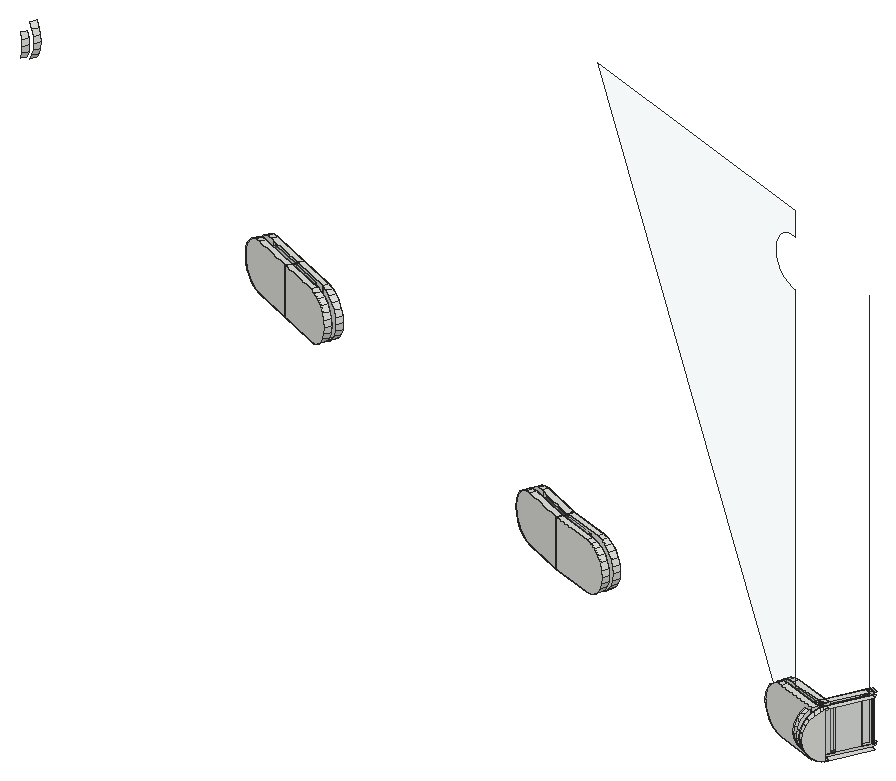
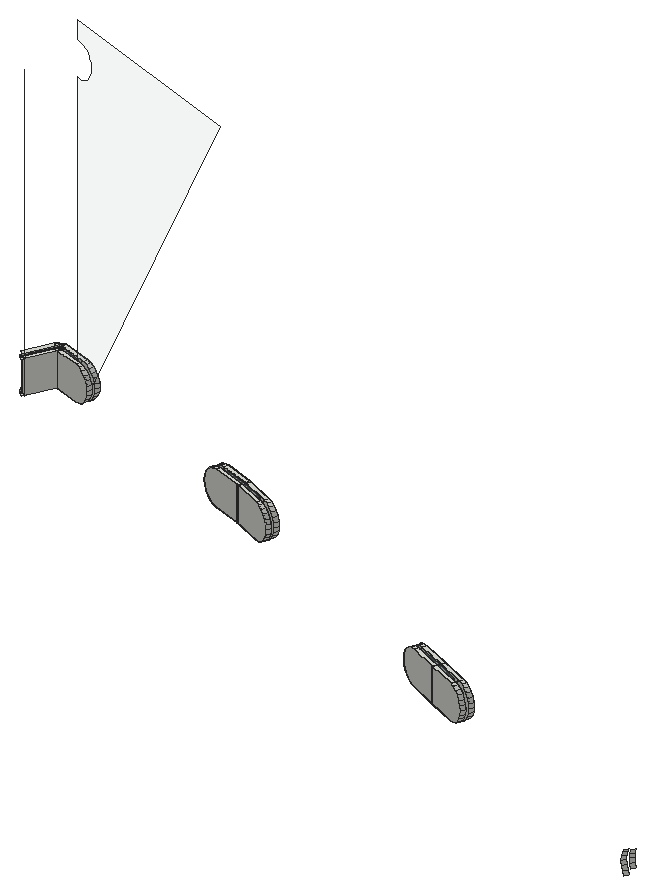
# SketchUp Ruby script. Lengths in inches.
U = 1.inch
M = Sketchup.active_model
def pt(a) = Geom::Point3d.new(a.map { |v| v * U })
def face(e, loops, mat)
  f = e.add_face(loops[0].map { |a| pt(a) })
  loops[1..].each { |l| e.add_face(l.map { |a| pt(a) }).erase! }
  f.material = f.back_material = mat if mat
  f
end
# faces: each face lists its corners as indices into pts; further lists are holes
def faces(e, pts, list, mat = nil) = list.each { |f| face(e, (f[0].is_a?(Array) ? f : [f]).map { |l| l.map { |i| pts[i] } }, mat) }
# xy, xz, yz: faces in a plane at the given z, y or x. An outline is a flat list of corners, or four numbers for a rectangle; further outlines are holes
def ring(l) = l.size == 4 ? [[l[0], l[1]], [l[2], l[1]], [l[2], l[3]], [l[0], l[3]]] : l.each_slice(2).to_a
def flat(e, list, mat, &to3) = list.each { |f| face(e, (f[0].is_a?(Array) ? f : [f]).map { |l| ring(l).map { |u, v| to3.(u, v) } }, mat) }
def xy(e, z, list, mat = nil) = flat(e, list, mat) { |x, y| [x, y, z] }
def xz(e, y, list, mat = nil) = flat(e, list, mat) { |x, z| [x, y, z] }
def yz(e, x, list, mat = nil) = flat(e, list, mat) { |y, z| [x, y, z] }
def lines(e, pts, list) = list.each { |a, b| e.add_line(pt(pts[a]), pt(pts[b])) }
# prism: a flat outline (further loops are holes) pulled along v
def prism(e, loops, v, mat = nil)
  f = face(e, loops, mat); d = Geom::Vector3d.new(v.map { |x| x * U })
  f.pushpull(f.normal.samedirection?(d) ? d.length : -d.length)
end
def box(e, o, s, mat = nil) = prism(e, [[o, [o[0] + s[0], o[1], o[2]], [o[0] + s[0], o[1] + s[1], o[2]], [o[0], o[1] + s[1], o[2]]]], [0, 0, s[2]], mat)
def at(x, y, z, deg = 0) = Geom::Transformation.translation(pt([x, y, z])) * Geom::Transformation.rotation(ORIGIN, Z_AXIS, deg.degrees)
def axes(o, x, y, z) = Geom::Transformation.new([*x, 0, *y, 0, *z, 0, *pt(o).to_a, 1])
def part(name) = M.definitions.add(name)
# library, detail: a bought-in or finely detailed component or shape, given as its bounding box
def library(name, o, s) = part(name).tap { |d| box(d.entities, o, s) }
def detail(e, o, s) = box(e.add_group.entities, o, s)
def put(e, d, t, mat = nil) = e.add_instance(d, t).tap { |i| i.material = mat if mat }
def group(e, t, mat = nil) = e.add_group.tap { |g| g.transformation = t; g.material = mat if mat }.entities
root = M.entities
M.materials.add("Glass_Safety_01").color = [204, 235, 244]
M.materials["Glass_Safety_01"].alpha = 0.1
xy(root,333,[[842.969,535.471,841.097,536.081,841.182,536.343,841.404,536.271,843.054,535.733],[843.42,535.662,843.173,535.784,843.242,535.924,843.489,535.803],[843.489,535.803,843.242,535.924,844.039,537.551,844.286,537.43],[842.996,535.87,842.749,535.992,842.769,536.033,843.034,535.947,843.115,535.921,843.2,536.183,843.156,536.197,842.891,536.283,843.615,537.759,843.862,537.638,843.156,536.197,843.065,536.011,843.034,535.947],[843.115,535.921,843.034,535.947,843.065,536.011,843.156,536.197,843.2,536.183],
  [843.034,535.947,842.769,536.033,842.817,536.132,843.065,536.011],[843.065,536.011,842.817,536.132,842.891,536.283,843.156,536.197],[842.769,536.033,841.465,536.458,841.243,536.53,841.329,536.792,842.891,536.283,842.817,536.132],[843.862,537.638,843.615,537.759,843.677,537.885,843.929,537.775,843.867,537.648],[843.929,537.775,843.677,537.885,843.68,537.892,843.684,537.9,843.931,537.779],
  [829.024,540.014,827.152,540.623,827.238,540.885,829.109,540.276],[829.17,540.463,827.307,541.069,827.417,541.322,827.401,541.329,829.256,540.725],[827.119,540.636,825.314,541.422,825.424,541.675,825.595,541.6,827.229,540.889],[827.307,541.069,827.299,541.073,827.384,541.335,827.401,541.329,827.417,541.322],[827.299,541.073,825.674,541.78,825.503,541.855,825.613,542.108,827.401,541.329,827.384,541.335],
  [809.928,548.122,808.124,548.907,808.234,549.16,810.038,548.374],[810.117,548.555,808.312,549.341,808.422,549.593,810.227,548.807],[808.124,548.907,806.319,549.693,806.429,549.946,806.582,549.879,808.234,549.16],[808.312,549.341,806.661,550.06,806.507,550.127,806.617,550.379,808.422,549.593]])
xy(root,333.078,[[843.054,535.733,841.557,536.221,841.618,536.408,843.034,535.947,842.996,535.87,843.084,535.827],[843.173,535.784,843.084,535.827,843.115,535.921,843.034,535.947,843.238,536.364,843.415,536.278],[843.084,535.827,842.996,535.87,843.034,535.947,843.115,535.921],[843.415,536.278,843.238,536.364,843.689,537.285,843.866,537.198],[828.735,540.398,827.238,540.885,827.268,540.979,827.307,541.069,828.796,540.585],
  [827.229,540.889,825.785,541.517,825.864,541.698,827.299,541.073,827.268,540.979],[827.268,540.979,827.299,541.073,827.307,541.069],[809.677,548.531,808.234,549.16,808.312,549.341,809.756,548.712],[808.234,549.16,806.79,549.789,806.868,549.969,808.312,549.341]],"Glass_Safety_01")
xy(root,335.047,[[843.054,535.733,843.084,535.827,842.996,535.87,843.034,535.947,841.618,536.408,841.557,536.221],[843.173,535.784,843.415,536.278,843.238,536.364,843.034,535.947,843.115,535.921,843.084,535.827],[843.084,535.827,843.115,535.921,843.034,535.947,842.996,535.87],[843.415,536.278,843.866,537.198,843.689,537.285,843.238,536.364],[828.735,540.398,828.796,540.585,827.307,541.069,827.268,540.979,827.238,540.885],
  [827.229,540.889,827.268,540.979,827.299,541.073,825.864,541.698,825.785,541.517],[827.268,540.979,827.307,541.069,827.299,541.073],[809.677,548.531,809.756,548.712,808.312,549.341,808.234,549.16],[808.234,549.16,808.312,549.341,806.868,549.969,806.79,549.789]],"Glass_Safety_01")
xy(root,335.126,[[842.969,535.471,843.054,535.733,841.404,536.271,841.182,536.343,841.097,536.081],[843.42,535.662,843.489,535.803,843.242,535.924,843.173,535.784],[843.489,535.803,844.286,537.43,844.039,537.551,843.242,535.924],[842.996,535.87,843.034,535.947,843.065,536.011,843.156,536.197,843.862,537.638,843.615,537.759,842.891,536.283,843.156,536.197,843.2,536.183,843.115,535.921,843.034,535.947,842.769,536.033,842.749,535.992],[843.115,535.921,843.2,536.183,843.156,536.197,843.065,536.011,843.034,535.947],
  [843.034,535.947,843.065,536.011,842.817,536.132,842.769,536.033],[843.065,536.011,843.156,536.197,842.891,536.283,842.817,536.132],[842.769,536.033,842.817,536.132,842.891,536.283,841.329,536.792,841.243,536.53,841.465,536.458],[843.862,537.638,843.867,537.647,843.867,537.648,843.929,537.775,843.677,537.885,843.615,537.759],[843.929,537.775,843.931,537.779,843.684,537.9,843.68,537.892,843.677,537.885],
  [829.024,540.014,829.109,540.276,827.238,540.885,827.152,540.623],[829.17,540.463,829.256,540.725,827.401,541.329,827.417,541.322,827.307,541.069],[827.119,540.636,827.229,540.889,825.595,541.6,825.424,541.675,825.314,541.422],[827.307,541.069,827.417,541.322,827.401,541.329,827.384,541.335,827.299,541.073],[827.299,541.073,827.384,541.335,827.401,541.329,825.613,542.108,825.503,541.855,825.674,541.78],
  [809.928,548.122,810.038,548.374,808.234,549.16,808.124,548.907],[810.117,548.555,810.227,548.807,808.422,549.593,808.312,549.341],[808.124,548.907,808.234,549.16,806.582,549.879,806.429,549.946,806.319,549.693],[808.312,549.341,808.422,549.593,806.617,550.379,806.507,550.127,806.661,550.06]])
p = [[843.368,535.556,333.036],[843.42,535.662,333.02],[843.42,535.662,335.105],[843.368,535.556,335.089],[843.255,535.326,334.983],[843.158,535.128,334.814],
  [843.084,534.976,334.594],[843.037,534.881,334.338],[843.021,534.848,334.0625],[843.037,534.881,333.787],[843.084,534.976,333.531],[843.158,535.128,333.311],
  [843.255,535.326,333.142],[843.121,535.677,335.089],[843.173,535.784,335.105],[843.173,535.784,335.047],[843.173,535.784,333.078],[843.173,535.784,333.02],
  [843.121,535.677,333.036],[843.008,535.447,333.142],[842.911,535.249,333.311],[842.837,535.098,333.531],[842.79,535.002,333.787],[842.774,534.97,334.0625],
  [842.79,535.002,334.338],[842.837,535.098,334.594],[842.911,535.249,334.814],[843.008,535.447,334.983],[843.862,537.638,333],[843.867,537.648,333],
  [843.929,537.775,333],[843.929,537.775,333.02],[843.929,537.775,333.078],[843.929,537.775,335.047],[843.929,537.775,335.106],[843.929,537.775,335.126],
  [843.867,537.648,335.126],[843.867,537.647,335.126],[843.862,537.638,335.126],[843.156,536.197,335.126],[843.065,536.011,335.126],[842.996,535.87,335.105],
  [842.944,535.764,335.089],[842.831,535.534,334.983],[842.734,535.336,334.814],[842.66,535.184,334.594],[842.613,535.089,334.338],[842.597,535.056,334.0625],
  [842.613,535.089,333.787],[842.66,535.184,333.531],[842.734,535.336,333.311],[842.831,535.534,333.142],[842.944,535.764,333.036],[842.996,535.87,333.02],
  [843.065,536.011,333],[843.156,536.197,333],[842.696,535.885,335.089],[842.749,535.992,335.105],[842.749,535.992,333.02],[842.696,535.885,333.036],
  [842.584,535.655,333.142],[842.487,535.457,333.311],[842.412,535.305,333.531],[842.366,535.21,333.787],[842.35,535.178,334.0625],[842.366,535.21,334.338],
  [842.412,535.305,334.594],[842.487,535.457,334.814],[842.584,535.655,334.983],[842.969,535.471,335.126],[841.097,536.081,335.126],[840.835,536.166,335.089],
  [840.592,536.246,334.983],[840.382,536.314,334.814],[840.222,536.366,334.594],[840.121,536.399,334.338],[840.086,536.41,334.0625],[840.121,536.399,333.787],
  [840.222,536.366,333.531],[840.382,536.314,333.311],[840.592,536.246,333.142],[840.835,536.166,333.036],[841.097,536.081,333],[842.969,535.471,333],
  [843.054,535.733,333],[843.054,535.733,333.078],[843.054,535.733,335.047],[843.054,535.733,335.126],[843.242,535.924,333],[843.489,535.803,333],
  [841.404,536.271,333],[841.404,536.271,335.126],[841.557,536.221,335.047],[841.557,536.221,333.078],[843.173,535.784,333],[843.42,535.662,333],
  [843.42,535.662,335.126],[843.173,535.784,335.126],[842.817,536.132,333],[843.415,536.278,333.078],[843.415,536.278,335.047],[843.242,535.924,335.126],
  [844.039,537.551,335.126],[844.04,537.553,335.125],[844.044,537.562,335.126],[844.044,537.562,335.124],[844.04,537.553,335.047],[844.044,537.562,335.047],
  [844.108,537.692,335.105],[844.108,537.692,335.047],[844.044,537.562,333.078],[844.108,537.692,333.078],[844.108,537.692,333.02],[844.044,537.562,333.001],
  [844.044,537.562,333],[844.039,537.551,333],[843.866,537.198,333.078],[844.039,537.552,333.078],[844.039,537.551,335.047],[843.866,537.198,335.047],
  [842.769,536.033,335.126],[841.465,536.458,335.126],[841.465,536.458,333],[842.769,536.033,333],[843.034,535.947,333],[843.115,535.921,333],
  [843.115,535.921,333.078],[843.034,535.947,333.078],[841.618,536.408,333.078],[841.618,536.408,335.047],[843.034,535.947,335.047],[843.115,535.921,335.047],
  [843.115,535.921,335.126],[843.034,535.947,335.126],[842.996,535.87,333],[842.996,535.87,333.078],[842.996,535.87,335.047],[842.996,535.87,335.126],
  [842.749,535.992,335.126],[842.749,535.992,333],[843.862,537.638,333.078],[843.689,537.285,333.078],[843.238,536.364,333.078],[843.931,537.779,333.02],
  [843.931,537.779,333.078],[843.931,537.779,335.047],[843.931,537.779,335.105],[843.867,537.648,335.124],[843.867,537.647,335.124],[843.862,537.638,335.047],
  [843.689,537.285,335.047],[843.238,536.364,335.047],[843.867,537.648,333.001],[843.2,536.183,333],[843.2,536.183,335.126],[843.615,537.759,335.126],
  [843.676,537.885,335.107],[843.676,537.885,333.018],[843.615,537.759,333],[842.891,536.283,333],[842.817,536.132,335.126],[842.891,536.283,335.126],
  [840.921,536.428,333.036],[841.182,536.343,333],[841.329,536.792,333],[841.067,536.878,333.036],[840.823,536.957,333.142],[840.614,537.025,333.311],
  [840.453,537.077,333.531],[840.352,537.11,333.787],[840.318,537.122,334.0625],[840.352,537.11,334.338],[840.453,537.077,334.594],[840.614,537.025,334.814],
  [840.823,536.957,334.983],[841.067,536.878,335.089],[841.329,536.792,335.126],[840.677,536.508,333.142],[841.182,536.343,335.126],[840.468,536.576,333.311],
  [840.307,536.628,333.531],[840.206,536.661,333.787],[840.172,536.672,334.0625],[840.206,536.661,334.338],[840.307,536.628,334.594],[840.468,536.576,334.814],
  [840.677,536.508,334.983],[840.921,536.428,335.089],[840.243,536.856,334.145],[840.804,536.674,333.113],[840.982,536.616,333.036],[841.243,536.53,333],
  [841.243,536.53,335.126],[840.982,536.616,335.089],[840.738,536.695,334.983],[840.529,536.763,334.814],[840.368,536.815,334.594],[840.267,536.848,334.338],
  [840.738,536.695,333.142],[843.983,537.885,333.036],[843.684,537.9,333.02],[843.736,538.006,333.036],[843.677,537.885,333],[843.677,537.885,335.126],
  [843.931,537.779,333],[843.684,537.9,333],[843.684,537.9,335.105],[843.684,537.9,335.126],[843.931,537.779,335.126],[843.68,537.892,333],
  [829.024,540.014,335.126],[827.152,540.623,335.126],[827.152,540.623,333],[829.024,540.014,333],[829.286,539.928,333.036],[829.529,539.849,333.142],
  [829.739,539.781,333.311],[829.899,539.729,333.531],[830,539.696,333.787],[830.035,539.684,334.0625],[830,539.696,334.338],[829.899,539.729,334.594],
  [829.739,539.781,334.814],[829.529,539.849,334.983],[829.286,539.928,335.089],[829.371,540.19,333.036],[829.615,540.111,333.142],[829.109,540.276,333],
  [829.109,540.276,335.126],[829.824,540.043,333.311],[829.985,539.991,333.531],[830.086,539.958,333.787],[830.12,539.946,334.0625],[830.086,539.958,334.338],
  [829.985,539.991,334.594],[829.824,540.043,334.814],[829.615,540.111,334.983],[829.371,540.19,335.089],[827.307,541.069,335.126],[827.299,541.073,335.126],
  [827.299,541.073,335.047],[827.299,541.073,333.078],[827.299,541.073,333],[827.307,541.069,333],[829.17,540.463,333],[829.432,540.378,333.036],
  [829.676,540.298,333.142],[829.885,540.23,333.311],[830.046,540.178,333.531],[830.147,540.145,333.787],[830.181,540.134,334.0625],[830.147,540.145,334.338],
  [830.046,540.178,334.594],[829.885,540.23,334.814],[829.676,540.298,334.983],[829.432,540.378,335.089],[829.17,540.463,335.126],[827.238,540.885,335.126],
  [827.238,540.885,333],[827.238,540.885,333.078],[828.735,540.398,333.078],[828.735,540.398,335.047],[827.238,540.885,335.047],[829.517,540.64,333.036],
  [829.761,540.56,333.142],[827.384,541.335,335.126],[827.401,541.329,335.126],[829.256,540.725,335.126],[829.517,540.64,335.089],[829.761,540.56,334.983],
  [829.97,540.492,334.814],[830.131,540.44,334.594],[830.232,540.407,334.338],[830.266,540.396,334.0625],[830.232,540.407,333.787],[830.131,540.44,333.531],
  [829.97,540.492,333.311],[829.256,540.725,333],[827.401,541.329,333],[827.384,541.335,333],[827.119,540.636,335.126],[825.314,541.422,335.126],
  [825.062,541.532,335.089],[824.827,541.634,334.983],[824.625,541.722,334.814],[824.47,541.789,334.594],[824.373,541.832,334.338],[824.339,541.846,334.0625],
  [824.373,541.832,333.787],[824.47,541.789,333.531],[824.625,541.722,333.311],[824.827,541.634,333.142],[825.062,541.532,333.036],[825.314,541.422,333],
  [827.119,540.636,333],[827.229,540.889,333],[827.229,540.889,333.078],[827.229,540.889,335.047],[827.229,540.889,335.126],[825.595,541.6,333],
  [825.595,541.6,335.126],[825.785,541.517,335.047],[825.785,541.517,333.078],[825.864,541.698,333.078],[825.864,541.698,335.047],[825.674,541.78,335.126],
  [825.674,541.78,333],[827.307,541.069,333.078],[827.307,541.069,335.047],[827.417,541.322,333],[827.417,541.322,335.126],[825.613,542.108,333],
  [825.36,542.218,333.036],[825.125,542.32,333.142],[824.923,542.408,333.311],[824.769,542.475,333.531],[824.671,542.518,333.787],[824.638,542.532,334.0625],
  [824.671,542.518,334.338],[824.769,542.475,334.594],[824.923,542.408,334.814],[825.125,542.32,334.983],[825.36,542.218,335.089],[825.613,542.108,335.126],
  [825.172,541.784,333.036],[825.424,541.675,333],[824.937,541.887,333.142],[825.424,541.675,335.126],[824.735,541.975,333.311],[824.58,542.042,333.531],
  [824.483,542.085,333.787],[824.449,542.099,334.0625],[824.483,542.085,334.338],[824.58,542.042,334.594],[824.735,541.975,334.814],[824.937,541.887,334.983],
  [825.172,541.784,335.089],[825.503,541.855,333],[825.503,541.855,335.126],[825.25,541.965,335.089],[825.015,542.067,334.983],[824.813,542.155,334.814],
  [824.659,542.223,334.594],[824.561,542.265,334.338],[824.528,542.279,334.0625],[824.561,542.265,333.787],[824.659,542.223,333.531],[824.813,542.155,333.311],
  [825.015,542.067,333.142],[825.25,541.965,333.036],[809.928,548.122,335.126],[808.124,548.907,335.126],[808.124,548.907,333],[809.928,548.122,333],
  [810.181,548.012,333.036],[810.416,547.909,333.142],[810.618,547.821,333.311],[810.772,547.754,333.531],[810.87,547.712,333.787],[810.903,547.697,334.0625],
  [810.87,547.712,334.338],[810.772,547.754,334.594],[810.618,547.821,334.814],[810.416,547.909,334.983],[810.181,548.012,335.089],[810.038,548.374,335.126],
  [810.038,548.374,333],[810.291,548.264,333.036],[810.526,548.162,333.142],[810.728,548.074,333.311],[810.882,548.007,333.531],[810.98,547.964,333.787],
  [811.013,547.95,334.0625],[810.98,547.964,334.338],[810.882,548.007,334.594],[810.728,548.074,334.814],[810.526,548.162,334.983],[810.291,548.264,335.089],
  [810.117,548.555,333],[810.117,548.555,335.126],[810.369,548.445,335.089],[810.604,548.342,334.983],[810.806,548.255,334.814],[810.961,548.187,334.594],
  [811.058,548.145,334.338],[811.092,548.13,334.0625],[811.058,548.145,333.787],[810.961,548.187,333.531],[810.806,548.255,333.311],[810.604,548.342,333.142],
  [810.369,548.445,333.036],[810.479,548.698,333.036],[810.714,548.595,333.142],[808.234,549.16,335.126],[808.234,549.16,333],[808.234,549.16,333.078],
  [809.677,548.531,333.078],[809.677,548.531,335.047],[808.234,549.16,335.047],[808.422,549.593,335.126],[810.227,548.807,335.126],[810.479,548.698,335.089],
  [810.714,548.595,334.983],[810.916,548.507,334.814],[811.071,548.44,334.594],[811.168,548.397,334.338],[811.202,548.383,334.0625],[811.168,548.397,333.787],
  [811.071,548.44,333.531],[810.916,548.507,333.311],[810.227,548.807,333],[808.422,549.593,333],[808.312,549.341,333],[808.312,549.341,335.126],
  [808.312,549.341,335.047],[809.756,548.712,335.047],[809.756,548.712,333.078],[808.312,549.341,333.078],[806.319,549.693,335.126],[806.067,549.803,335.089],
  [805.831,549.906,334.983],[805.63,549.994,334.814],[805.475,550.061,334.594],[805.377,550.103,334.338],[805.344,550.118,334.0625],[805.377,550.103,333.787],
  [805.475,550.061,333.531],[805.63,549.994,333.311],[805.831,549.906,333.142],[806.067,549.803,333.036],[806.319,549.693,333],[806.582,549.879,333],
  [806.582,549.879,335.126],[806.79,549.789,335.047],[806.79,549.789,333.078],[806.661,550.06,335.126],[806.661,550.06,333],[806.868,549.969,333.078],
  [806.868,549.969,335.047],[806.617,550.379,335.126],[806.617,550.379,333],[806.365,550.489,333.036],[806.13,550.591,333.142],[805.928,550.679,333.311],
  [805.773,550.747,333.531],[805.676,550.789,333.787],[805.643,550.804,334.0625],[805.676,550.789,334.338],[805.773,550.747,334.594],[805.928,550.679,334.814],
  [806.13,550.591,334.983],[806.365,550.489,335.089],[806.177,550.056,333.036],[806.429,549.946,333],[805.942,550.158,333.142],[806.429,549.946,335.126],
  [805.74,550.246,333.311],[805.585,550.314,333.531],[805.487,550.356,333.787],[805.454,550.371,334.0625],[805.487,550.356,334.338],[805.585,550.314,334.594],
  [805.74,550.246,334.814],[805.942,550.158,334.983],[806.177,550.056,335.089],[806.507,550.127,333],[806.507,550.127,335.126],[806.255,550.236,335.089],
  [806.02,550.339,334.983],[805.818,550.427,334.814],[805.663,550.494,334.594],[805.566,550.537,334.338],[805.533,550.551,334.0625],[805.566,550.537,333.787],
  [805.663,550.494,333.531],[805.818,550.427,333.311],[806.02,550.339,333.142],[806.255,550.236,333.036],[843.084,535.827,333.078],[843.084,535.827,335.047],
  [840.233,536.86,334.0625],[840.267,536.848,333.787],[840.368,536.815,333.531],[840.529,536.763,333.311],[843.867,537.648,333.078],[843.867,537.647,335.047],
  [828.796,540.585,333.078],[828.796,540.585,335.047],[827.268,540.979,333.078],[827.268,540.979,335.047],[827.303,541.071,335.047],[827.303,541.071,333.078],
  [789.74,557.429,333.531],[789.586,557.497,333.311],[789.696,557.749,333.311],[789.85,557.682,333.531],[789.662,557.249,333.531],[789.759,557.206,333.787],
  [789.649,556.954,333.787],[789.552,556.996,333.531],[789.838,557.387,333.787],[789.948,557.639,333.787],[789.792,557.192,334.0625],[789.682,556.939,334.0625],
  [789.871,557.372,334.0625],[789.981,557.625,334.0625],[841.465,536.458,351.283],[829.17,540.463,354.511],[841.465,536.458,354.511],[841.465,536.458,353.409],
  [841.243,536.53,353.409],[840.982,536.616,353.373],[840.738,536.695,353.267],[840.529,536.763,353.098],[840.368,536.815,352.877],[840.267,536.848,352.621],
  [840.233,536.86,352.346],[840.267,536.848,352.071],[840.368,536.815,351.815],[840.529,536.763,351.594],[840.738,536.695,351.425],[840.982,536.616,351.319],
  [841.243,536.53,351.283],[789.759,557.206,334.338],[789.649,556.954,334.338],[789.838,557.387,334.338],[789.948,557.639,334.338],[789.662,557.249,334.594],
  [789.552,556.996,334.594],[789.74,557.429,334.594],[789.85,557.682,334.594],[789.586,557.497,334.814],[789.696,557.749,334.814],[843.489,535.803,335.126],
  [843.983,537.885,335.089],[843.736,538.006,335.089],[843.862,537.638,351.283],[843.862,537.638,351.362],[843.863,537.64,351.362],[843.863,537.64,351.283],
  [843.68,537.892,335.126]]
faces(root,p,[[0,1,2,3,4,5,6,7,8,9,10,11,12],[13,14,15,16,17,18,19,20,21,22,23,24,25,26,27],[28,29,30,31,32,33,34,35,36,37,38,39,40,41,42,43,44,45,46,47,48,49,50,51,52,53,54,55],[56,57,58,59,60,61,62,63,64,65,66,67,68],[19,18,0,12],[69,70,71,72,73,74,75,76,77,78,79,80,81,82,83],[52,51,60,59],[84,85,86,87,69,83],
  [18,17,88,89,1,0],[84,90,91,87,86,92,93,85],[17,94,95,1,2,96,97,14,15,16],[95,89,1],[53,52,59,58,98,54],[94,17,88],[[88,17,16,99,100,15,14,101,102,103,104,105,103,106,107,105,108,109,107,110,111,112,113,114,115],[116,117,118,119]],[120,121,122,123,124,125,126,127,128,129,130,131,132,133],
  [134,53,135,136,41,137,138,57,58,139],[124,54,53,134],[55,28,140,141,142,127,135,53,54],[31,143,144,145,146,34,147,148,38,149,150,151,130,136,135,127,142,141,140,28,152],[126,125,153,154,132,131],[139,58,98,123],[155,156,157,158,159,98,58,57,160,161],[162,163,82,81],
  [39,154,153,55,159,164,165,166,167,168,169,170,171,172,173,174,175,176,161],[177,162,81,80],[178,91,90,163,162,177,179,180,181,182,183,184,185,186,187],[191,190,165,164],[189,198,166,165,190],[199,143,31,152,28,158,157,200,201],[158,157,202],[30,31,32,33,34,35,203,156,157,202],
  [143,204,205,200,206,207,208,146,145,144],[200,157,156,206],[209,202,157,200,205],[210,211,212,213,214,215,216,217,218,219,220,221,222,223,224],[225,226,215,214],[227,225,214,213],[238,239,240,241,242,243,244,245,246,247,248,249,250,251,252,253,254,255,256],[257,228,227,258,259,260,261,262],
  [246,245,263,264],[265,266,267,268,269,270,271,272,273,274,275,276,264,263,277,278,279],[245,244,277,263],[280,281,282,283,284,285,286,287,288,289,290,291,292,293,294],[295,296,297,298,280,294],[259,258,212,211,257,262],[295,299,300,298,297,301,302,296],[242,241,303,304,240,239,305,306],
  [238,239,240,241,242,243,307,308],[242,241,240,239,265,279],[307,243,309,310,238,308],[266,310,309,278,311,312,313,314,315,316,317,318,319,320,321,322,323],[324,325,293,292],[326,324,292,291],[327,300,299,325,324,326,328,329,330,331,332,333,334,335,336],[337,306,305,338,339,340,341,342,343,344,345,346,347,348,349],
  [337,349,312,311],[349,348,313,312],[350,351,352,353,354,355,356,357,358,359,360,361,362,363,364],[367,368,355,354],[366,367,354,353],[389,390,391,392],[393,365,366,394,395,396,397,398],[399,400,401,402,403,404,405,406,407,408,409,392,391,410,411],
  [390,378,410,391],[412,378,379,413,414,415,416,417],[351,418,419,420,421,422,423,424,425,426,427,428,429,430,352],[394,395,398,393,351,352],[394,431,432,393,398,433,434,395],[413,435,436,412,417,437,438,414],[417,412,411,399,413,414],[439,399,411,440,441,442,443,444,445,446,447,448,449,450,451],
  [452,453,430,429],[454,452,429,428],[455,432,431,453,452,454,456,457,458,459,460,461,462,463,464],[465,436,435,466,467,468,469,470,471,472,473,474,475,476,477],[465,477,441,440],[477,476,442,441],[20,19,12,11],[51,50,61,60],
  [179,177,80,79],[188,480,481,482,483,198,189],[198,483,167,166],[226,229,216,215],[247,246,264,276],[328,326,291,290],[348,347,314,313],[368,369,356,355],
  [388,389,392,409],[456,454,428,427],[476,475,443,442],[21,20,11,10],[50,49,62,61],[180,179,79,78],[483,482,168,167],[229,230,217,216],
  [248,247,276,275],[329,328,290,289],[347,346,315,314],[369,370,357,356],[387,388,409,408],[457,456,427,426],[475,474,444,443],[492,493,494,495],
  [22,21,10,9],[49,48,63,62],[181,180,78,77],[482,481,169,168],[230,231,218,217],[249,248,275,274],[330,329,289,288],[346,345,316,315],
  [370,371,358,357],[386,387,408,407],[458,457,426,425],[474,473,445,444],[496,497,498,499],[500,492,495,501],[23,22,9,8],[48,47,64,63],
  [182,181,77,76],[481,480,170,169],[231,232,219,218],[250,249,274,273],[331,330,288,287],[345,344,317,316],[371,372,359,358],[385,386,407,406],
  [459,458,425,424],[473,472,446,445],[497,502,503,498],[504,500,501,505],[24,23,8,7],[47,46,65,64],[183,182,76,75],[188,197,171,170,480],
  [232,233,220,219],[251,250,273,272],[332,331,287,286],[344,343,318,317],[372,373,360,359],[384,385,406,405],[460,459,424,423],[472,471,447,446],
  [502,523,524,503],[525,504,505,526],[25,24,7,6],[46,45,66,65],[184,183,75,74],[197,196,172,171],[233,234,221,220],[252,251,272,271],
  [333,332,286,285],[343,342,319,318],[373,374,361,360],[383,384,405,404],[461,460,423,422],[471,470,448,447],[523,527,528,524],[529,525,526,530],
  [26,25,6,5],[45,44,67,66],[185,184,74,73],[196,195,173,172],[234,235,222,221],[253,252,271,270],[334,333,285,284],[342,341,320,319],
  [374,375,362,361],[382,383,404,403],[462,461,422,421],[470,469,449,448],[531,529,530,532],[27,26,5,4],[44,43,68,67],[186,185,73,72],
  [195,194,174,173],[235,236,223,222],[254,253,270,269],[335,334,284,283],[341,340,321,320],[375,376,363,362],[381,382,403,402],[463,462,421,420],
  [469,468,450,449],[13,27,4,3],[43,42,56,68],[41,136,130,151,150,149,38,39,40],[187,186,72,71],[194,193,175,174],[236,237,224,223],[255,254,269,268],
  [336,335,283,282],[340,339,322,321],[376,377,364,363],[380,381,402,401],[464,463,420,419],[468,467,451,450],[101,14,13,3,2,533],[96,2,533],
  [41,40,160,57,56,42],[97,101,14],[137,41,40,133],[120,160,57,138],[178,187,71,70],[193,192,176,175],[38,148,147,34,146,534,535,206,156,155],[155,203,156],
  [206,156,203,540,207],[237,228,210,224],[256,255,268,267],[327,336,282,281],[339,338,323,322],[377,365,350,364],[379,380,401,400],[455,464,419,418],
  [467,466,439,451]])
faces(root,p,[[188,189,190,191,122,121,192,193,194,195,196,197],[228,227,225,226,229,230,231,232,233,234,235,236,237],[244,256,255,254,253,252,251,250,249,248,247,246,245],[365,366,367,368,369,370,371,372,373,374,375,376,377],[378,379,380,381,382,383,384,385,386,387,388,389,390],[85,93,92,86],[85,478,479,86],[478,479,136,135],
  [131,479,478,126],[479,478,16,15],[99,16,15,100],[127,126,131,130,129,128],[130,151,142,127,135,136],[93,92,129,128],[99,100,151,142],[99,116,119,100],
  [141,142,151,150],[116,141,150,119],[150,149,140,141],[484,140,149,485],[260,259,262,261],[260,486,487,261],[486,307,308,487],[296,302,301,297],
  [296,488,489,297],[489,488,259,262],[488,489,240,241],[308,489,488,307],[304,240,241,303],[490,308,307,491,241,240],[302,301,304,303],[396,395,398,397],
  [416,415,397,396],[417,416,415,414],[395,434,433,398],[395,417,414,398],[414,438,437,417],[434,433,438,437],[506,121,192,193,194,195,196,197,188,507,508,509,510,511,512,513,514,515,516,517,518,519,520,521,522],[149,38,148,485],
  [37,148,38,536,537,538,539]],"Glass_Safety_01")
